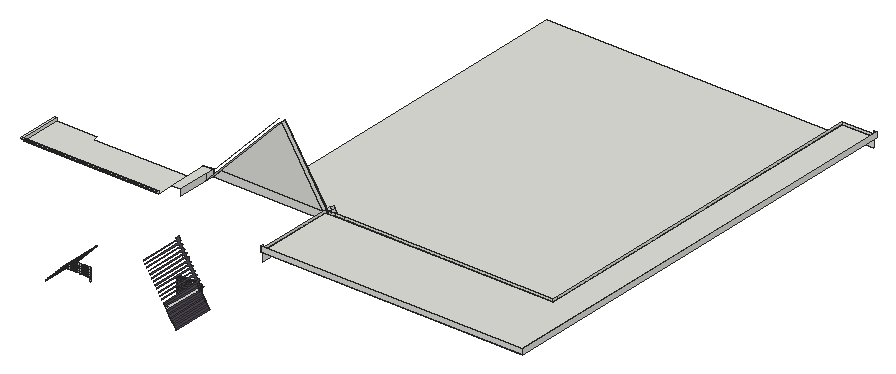
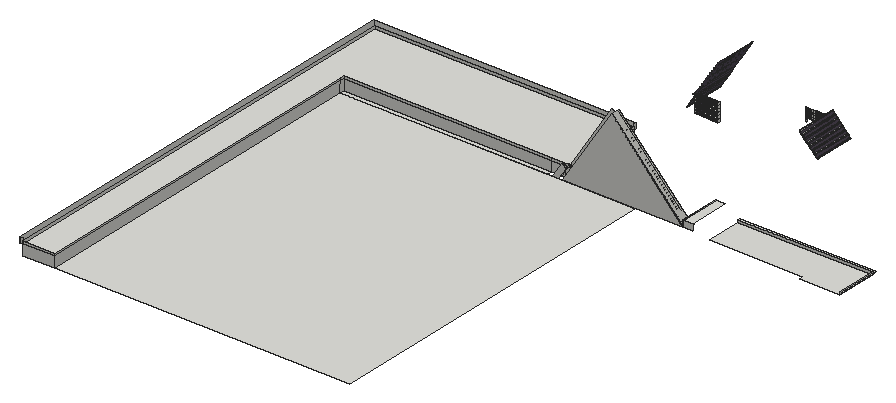
# SketchUp Ruby script. Lengths in inches.
U = 1.inch
M = Sketchup.active_model
def pt(a) = Geom::Point3d.new(a.map { |v| v * U })
def face(e, loops, mat)
  f = e.add_face(loops[0].map { |a| pt(a) })
  loops[1..].each { |l| e.add_face(l.map { |a| pt(a) }).erase! }
  f.material = f.back_material = mat if mat
  f
end
# faces: each face lists its corners as indices into pts; further lists are holes
def faces(e, pts, list, mat = nil) = list.each { |f| face(e, (f[0].is_a?(Array) ? f : [f]).map { |l| l.map { |i| pts[i] } }, mat) }
# xy, xz, yz: faces in a plane at the given z, y or x. An outline is a flat list of corners, or four numbers for a rectangle; further outlines are holes
def ring(l) = l.size == 4 ? [[l[0], l[1]], [l[2], l[1]], [l[2], l[3]], [l[0], l[3]]] : l.each_slice(2).to_a
def flat(e, list, mat, &to3) = list.each { |f| face(e, (f[0].is_a?(Array) ? f : [f]).map { |l| ring(l).map { |u, v| to3.(u, v) } }, mat) }
def xy(e, z, list, mat = nil) = flat(e, list, mat) { |x, y| [x, y, z] }
def xz(e, y, list, mat = nil) = flat(e, list, mat) { |x, z| [x, y, z] }
def yz(e, x, list, mat = nil) = flat(e, list, mat) { |y, z| [x, y, z] }
def lines(e, pts, list) = list.each { |a, b| e.add_line(pt(pts[a]), pt(pts[b])) }
# prism: a flat outline (further loops are holes) pulled along v
def prism(e, loops, v, mat = nil)
  f = face(e, loops, mat); d = Geom::Vector3d.new(v.map { |x| x * U })
  f.pushpull(f.normal.samedirection?(d) ? d.length : -d.length)
end
def box(e, o, s, mat = nil) = prism(e, [[o, [o[0] + s[0], o[1], o[2]], [o[0] + s[0], o[1] + s[1], o[2]], [o[0], o[1] + s[1], o[2]]]], [0, 0, s[2]], mat)
def at(x, y, z, deg = 0) = Geom::Transformation.translation(pt([x, y, z])) * Geom::Transformation.rotation(ORIGIN, Z_AXIS, deg.degrees)
def axes(o, x, y, z) = Geom::Transformation.new([*x, 0, *y, 0, *z, 0, *pt(o).to_a, 1])
def part(name) = M.definitions.add(name)
# library, detail: a bought-in or finely detailed component or shape, given as its bounding box
def library(name, o, s) = part(name).tap { |d| box(d.entities, o, s) }
def detail(e, o, s) = box(e.add_group.entities, o, s)
def put(e, d, t, mat = nil) = e.add_instance(d, t).tap { |i| i.material = mat if mat }
def group(e, t, mat = nil) = e.add_group.tap { |g| g.transformation = t; g.material = mat if mat }.entities
root = M.entities
M.materials.add("[Color M06]").color = [79, 71, 84]
xy(root,341.52,[[1096.79,2376.24,1127.76,2378.12]])
xy(root,341.93,[[1096.79,2376.24,1127.76,2378.12]])
xy(root,342.6875,[[771.375,2530.63,948.3125,2530.63,948.3125,2578.12,824.9375,2578.12,824.9375,2584.2,771.375,2584.2]])
xy(root,345.06,[[1096.79,2376.24,1127.76,2378.12]])
xy(root,346,[[1096.79,2376.24,1127.76,2378.12]])
xy(root,346.3125,[[768.8125,2528.07,771.375,2530.63],[771.375,2528.07,948.3125,2530.63],[768.8125,2530.63,771.375,2584.2]])
xy(root,349.12,[[1096.79,2376.24,1127.76,2378.12]])
xy(root,350.06,[[1096.79,2376.24,1127.76,2378.12]])
xy(root,350.1875,[[1156.15,2578.12,1429.3,2584.2],[1041.36,2584.2,1429.3,3053.87]])
xy(root,353.18,[[1096.79,2376.24,1127.76,2378.12]])
xy(root,354.12,[[1096.79,2376.24,1127.76,2378.12]])
xy(root,355.71,[[984.09,2332.13,986.27,2332.76],[986.875,2332.13,989.1875,2332.76],[989.79,2332.13,992.1,2332.76],[995.61,2332.13,997.92,2332.76],[1004.35,2332.13,1006.66,2332.76],
  [1007.26,2332.13,1009.57,2332.76],[1010.17,2332.13,1012.48,2332.76],[1013.08,2332.13,1015.4,2332.76],[1015.99,2332.13,1018.31,2332.76]])
xy(root,356.21,[[984.5625,2332.13,986.27,2332.76],[986.875,2332.13,989.1875,2332.76],[989.79,2332.13,992.1,2332.76],[992.7,2332.13,995.01,2332.76],[995.61,2332.13,997.92,2332.76],
  [998.52,2332.13,1000.83,2332.76],[1001.43,2332.13,1003.75,2332.76],[1004.35,2332.13,1006.66,2332.76],[1007.26,2332.13,1009.57,2332.76],[1010.17,2332.13,1012.48,2332.76],
  [1013.08,2332.13,1015.4,2332.76],[1015.99,2332.13,1018.31,2332.76]])
xy(root,357.25,[[1096.79,2376.24,1127.76,2378.12]])
xy(root,358.06,[[1096.79,2376.24,1127.76,2378.12]])
xy(root,358.5,[[965.61,2530.63,977.92,2584.2]])
xy(root,358.52,[[986.875,2332.13,989.1875,2332.76],[989.79,2332.13,992.1,2332.76],[992.7,2332.13,995.01,2332.76],[995.61,2332.13,997.92,2332.76],[998.52,2332.13,1000.83,2332.76],
  [1001.43,2332.13,1003.75,2332.76],[1004.35,2332.13,1006.66,2332.76],[1007.26,2332.13,1009.57,2332.76],[1010.17,2332.13,1012.48,2332.76],[1013.08,2332.13,1015.4,2332.76],
  [1015.99,2332.13,1018.31,2332.76]])
xy(root,359.02,[[987.2,2332.13,989.1875,2332.76],[989.79,2332.13,992.1,2332.76],[992.7,2332.13,995.01,2332.76],[995.61,2332.13,997.92,2332.76],[998.52,2332.13,1000.83,2332.76],
  [1001.43,2332.13,1003.75,2332.76],[1004.35,2332.13,1006.66,2332.76],[1007.26,2332.13,1009.57,2332.76],[1010.17,2332.13,1012.48,2332.76],[1013.08,2332.13,1015.4,2332.76],
  [1015.99,2332.13,1018.31,2332.76]])
xy(root,361.18,[[1096.79,2376.24,1127.76,2378.12]])
xy(root,361.34,[[989.79,2332.13,992.1,2332.76],[992.7,2332.13,995.01,2332.76],[995.61,2332.13,997.92,2332.76],[998.52,2332.13,1000.83,2332.76],[1001.43,2332.13,1003.75,2332.76],
  [1004.35,2332.13,1006.66,2332.76],[1007.26,2332.13,1009.57,2332.76],[1010.17,2332.13,1012.48,2332.76],[1013.08,2332.13,1015.4,2332.76],[1015.99,2332.13,1018.31,2332.76]])
xy(root,361.84,[[989.84,2332.13,992.1,2332.76],[992.7,2332.13,995.01,2332.76],[995.61,2332.13,997.92,2332.76],[998.52,2332.13,1000.83,2332.76],[1001.43,2332.13,1003.75,2332.76],
  [1004.35,2332.13,1006.66,2332.76],[1007.26,2332.13,1009.57,2332.76],[1010.17,2332.13,1012.48,2332.76],[1013.08,2332.13,1015.4,2332.76],[1015.99,2332.13,1018.31,2332.76]])
xy(root,362,[[1096.79,2376.24,1127.76,2378.12]])
xy(root,363.75,[[1130.09,2472.4,1470.74,2475.84],[1470.74,2472.4,1474.18,2475.84],[1130.09,2475.84,1130.09,2578.12,1429.3,2578.12,1429.3,3053.87,1470.74,3053.87,1470.74,2475.84],[1470.74,2475.84,1474.18,3053.87]])
xy(root,363.92,[[1127.76,2373.56,1129.63,2378.12]])
xy(root,364.15,[[992,2332.13,992.1,2332.76],[992.7,2332.13,995.01,2332.76],[995.61,2332.13,997.92,2332.76],[998.52,2332.13,1000.83,2332.76],[1001.43,2332.13,1003.75,2332.76],
  [1004.35,2332.13,1006.66,2332.76],[1007.26,2332.13,1009.57,2332.76],[1010.17,2332.13,1012.48,2332.76],[1013.08,2332.13,1015.4,2332.76],[1015.99,2332.13,1018.31,2332.76]])
xy(root,364.65,[[992.7,2332.13,995.01,2332.76],[995.61,2332.13,997.92,2332.76],[998.52,2332.13,1000.83,2332.76],[1001.43,2332.13,1003.75,2332.76],[1004.35,2332.13,1006.66,2332.76],
  [1007.26,2332.13,1009.57,2332.76],[1010.17,2332.13,1012.48,2332.76],[1013.08,2332.13,1015.4,2332.76],[1015.99,2332.13,1018.31,2332.76]])
xy(root,365.12,[[1096.79,2376.24,1126.98,2378.12]])
xz(root,2332.76,[[1015.99,350.59,1018.31,352.9],[1015.99,353.4,1018.31,355.71]])
xz(root,2371.68,[[1129.26,360.76,1129.63,360.99,1129.57,361.08,1129.21,360.85],[1128.57,361.83,1128.94,362.07,1127.76,363.92,1127.76,363.11],[1127.76,363.11,1127.39,363.68,1127.76,363.92],[1126.93,364.39,1126.88,364.48,1127.25,364.71,1127.3,364.625]])
xz(root,2373.56,[[970.79,341.69,973.21,344.27,972.75,344.7,970.33,342.125],[1140.21,343.68,1140.58,343.92,1138.88,346.56,1138.52,346.32],[974.08,345.2,976.51,347.77,976.05,348.2,973.63,345.63],[1137.88,347.3125,1138.25,347.55,1136.56,350.19,1136.1875,349.95],[977.38,348.7,979.8,351.28,979.35,351.7,976.93,349.13],
  [1135.56,350.94,1135.92,351.18,1134.23,353.82,1133.86,353.58],[980.68,352.21,983.1,354.78,982.65,355.21,980.23,352.64],[1133.23,354.57,1133.6,354.81,1131.9,357.45,1131.53,357.22],[983.98,355.71,986.4,358.28,985.95,358.71,983.53,356.14],[1130.9,358.2,1131.27,358.4375,1129.63,360.99,1129.63,360.18],
  [987.28,359.22,989.7,361.79,989.25,362.22,986.82,359.64],[1129.63,360.18,1129.26,360.76,1129.63,360.99],[1129.63,360.99,1129.63,363.92,1127.76,363.92,1128.94,362.07,1129.57,361.08],[990.58,362.72,993,365.29,992.54,365.72,990.12,363.15],[1127.39,363.68,1126.93,364.39,1127.3,364.625,1127.76,363.92],
  [1126.25,365.46,1124.61,368.02,1124.98,368.25,1126.61,365.7]])
xz(root,2376.24,[[1096.79,341.93,1127.76,345.06],[1096.79,346,1127.76,349.12],[1096.79,350.06,1127.76,353.18],[1096.79,354.12,1127.76,357.25],[1096.79,358.06,1127.76,361.18],
  [1096.79,362,1127.76,362,1127.76,363.92,1126.98,365.12,1096.79,365.12]],"[Color M06]")
xz(root,2378.12,[[1096.79,341.52,1127.76,341.93],[1096.79,345.06,1127.76,346],[1096.79,349.12,1127.76,350.06],[1096.79,353.18,1127.76,354.12],[1096.79,357.25,1127.76,358.06],
  [1096.79,361.18,1127.76,362],[1127.76,363.92,1127.76,365.12,1126.98,365.12],[1096.79,365.12,1126.98,365.12,1126.26,366.25,1096.79,366.25]])
xz(root,2472.4,[[1130.09,363.75,1474.18,370.8125]])
xz(root,2475.84,[[1130.09,363.75,1470.74,367.1875]])
xz(root,2530.63,[[771.375,342.6875,948.3125,346.3125]])
xz(root,2578.12,[[1130.09,350.1875,1130.09,360.28,1136.56,350.1875],[1136.56,350.1875,1136.56,359.1,1133.58,363.75,1130.09,363.75,1130.09,360.28],[1136.56,350.1875,1142.28,350.1875,1136.56,359.1],[1142.28,350.1875,1136.56,359.1,1136.56,363.75,1142.28,363.75],[1142.28,350.1875,1156.15,363.75],
  [1156.15,350.1875,1429.3,363.75],[1136.56,359.1,1133.58,363.75,1136.56,363.75],[1130.09,360.28,1130.09,364.9375,1127.1,364.9375],[1130.09,363.75,1130.09,364.9375,1132.82,364.9375,1133.58,363.75],[1133.58,363.75,1132.82,364.9375,1131.375,367.1875,1133.58,367.1875],
  [1133.58,363.75,1136.56,367.1875],[1136.56,363.75,1142.28,367.1875],[1142.28,363.75,1156.15,367.1875],[1156.15,363.75,1429.3,367.1875],[991.81,364.9375,1072.29,450.4375,1127.1,364.9375],
  [1127.1,364.9375,1072.29,450.4375,1076.34,453.03,1131.15,367.53,1130.61,367.1875,1130.09,367.1875,1130.09,366.85],[1127.1,364.9375,1130.09,366.85,1130.09,364.9375],[1130.09,364.9375,1130.09,366.85,1130.61,367.1875,1131.375,367.1875,1132.82,364.9375]])
xz(root,2583.74,[[965.61,357.04,964.88,357.73,965.61,358.5]])
xz(root,2584.2,[[1149.7,340.75,1153.99,343.5,1149.7,350.1875],[1142.28,341.27,1142.28,350.1875,1136.56,350.1875],[965.61,350.1875,977.92,358.5],[977.92,350.1875,1072.29,450.4375,1136.56,350.1875],[1142.28,350.1875,1132.82,364.9375,1138.08,368.3125,1149.7,350.1875],
  [1132.82,364.9375,1131.15,367.53,1136.41,370.91,1138.08,368.3125]])
xz(root,3053.87,[[1429.3,350.1875,1470.74,363.75],[1429.3,363.75,1470.74,367.1875],[1470.74,363.75,1474.18,370.8125]])
yz(root,771.375,[[2530.63,342.6875,2584.2,346.3125]])
yz(root,977.92,[[2530.63,350.1875,2571.59,358.5],[2571.59,350.1875,2583.74,358.5],[2583.74,350.1875,2584.2,358.5]])
yz(root,986.27,[[2332.13,356.21,2332.76,358.04]])
yz(root,986.875,[[2332.13,356.21,2332.76,358.52]])
yz(root,989.1875,[[2332.13,356.21,2332.76,358.52],[2332.13,359.02,2332.76,361.14]])
yz(root,989.79,[[2332.13,356.21,2332.76,358.52],[2332.13,359.02,2332.76,361.34]])
yz(root,992.1,[[2332.13,356.21,2332.76,358.52],[2332.13,359.02,2332.76,361.34],[2332.13,361.84,2332.76,364.15]])
yz(root,992.7,[[2332.13,356.21,2332.76,358.52],[2332.13,359.02,2332.76,361.34],[2332.13,361.84,2332.76,364.15],[2332.13,364.65,2332.76,364.89]])
yz(root,995.01,[[2332.13,356.21,2332.76,358.52],[2332.13,359.02,2332.76,361.34],[2332.13,361.84,2332.76,364.15],[2332.13,364.65,2332.76,366.96]])
yz(root,995.61,[[2332.13,356.21,2332.76,358.52],[2332.13,359.02,2332.76,361.34],[2332.13,361.84,2332.76,364.15],[2332.13,364.65,2332.76,366.96]])
yz(root,997.92,[[2332.13,356.21,2332.76,358.52],[2332.13,359.02,2332.76,361.34],[2332.13,361.84,2332.76,364.15],[2332.13,364.65,2332.76,366.96]])
yz(root,998.52,[[2332.13,356.21,2332.76,358.52],[2332.13,359.02,2332.76,361.34],[2332.13,361.84,2332.76,364.15],[2332.13,364.65,2332.76,366.96]])
yz(root,1000.83,[[2332.13,356.21,2332.76,358.52],[2332.13,359.02,2332.76,361.34],[2332.13,361.84,2332.76,364.15],[2332.13,364.65,2332.76,366.96]])
yz(root,1001.43,[[2332.13,356.21,2332.76,358.52],[2332.13,359.02,2332.76,361.34],[2332.13,361.84,2332.76,364.15],[2332.13,364.65,2332.76,366.96]])
yz(root,1003.75,[[2332.13,356.21,2332.76,358.52],[2332.13,359.02,2332.76,361.34],[2332.13,361.84,2332.76,364.15],[2332.13,364.65,2332.76,366.96]])
yz(root,1004.35,[[2332.13,356.21,2332.76,358.52],[2332.13,359.02,2332.76,361.34],[2332.13,361.84,2332.76,364.15],[2332.13,364.65,2332.76,366.96]])
yz(root,1006.66,[[2332.13,356.21,2332.76,358.52],[2332.13,359.02,2332.76,361.34],[2332.13,361.84,2332.76,364.15],[2332.13,364.65,2332.76,366.96]])
yz(root,1007.26,[[2332.13,356.21,2332.76,358.52],[2332.13,359.02,2332.76,361.34],[2332.13,361.84,2332.76,364.15],[2332.13,364.65,2332.76,366.96]])
yz(root,1009.57,[[2332.13,356.21,2332.76,358.52],[2332.13,359.02,2332.76,361.34],[2332.13,361.84,2332.76,364.15],[2332.13,364.65,2332.76,366.96]])
yz(root,1010.17,[[2332.13,356.21,2332.76,358.52],[2332.13,359.02,2332.76,361.34],[2332.13,361.84,2332.76,364.15],[2332.13,364.65,2332.76,366.96]])
yz(root,1012.48,[[2332.13,356.21,2332.76,358.52],[2332.13,359.02,2332.76,361.34],[2332.13,361.84,2332.76,364.15],[2332.13,364.65,2332.76,366.96]])
yz(root,1013.08,[[2332.13,356.21,2332.76,358.52],[2332.13,359.02,2332.76,361.34],[2332.13,361.84,2332.76,364.15],[2332.13,364.65,2332.76,366.96]])
yz(root,1015.4,[[2332.13,356.21,2332.76,358.52],[2332.13,359.02,2332.76,361.34],[2332.13,361.84,2332.76,364.15],[2332.13,364.65,2332.76,366.96]])
yz(root,1015.99,[[2332.13,356.21,2332.76,358.52],[2332.13,359.02,2332.76,361.34],[2332.13,361.84,2332.76,364.15],[2332.13,364.65,2332.76,366.96]])
yz(root,1018.31,[[2332.13,356.21,2332.76,358.52],[2332.13,359.02,2332.76,361.34],[2332.13,361.84,2332.76,364.15],[2332.13,364.65,2332.76,366.96]])
yz(root,1096.79,[[2376.24,341.93,2378.12,345.06],[2376.24,346,2378.12,349.12],[2376.24,350.06,2378.12,353.18],[2376.24,354.12,2378.12,357.25],[2376.24,358.06,2378.12,361.18],
  [2376.24,362,2378.12,365.12]])
yz(root,1127.76,[[2376.24,341.93,2378.12,345.06],[2376.24,346,2378.12,349.12],[2376.24,350.06,2378.12,353.18],[2376.24,354.12,2378.12,357.25],[2376.24,358.06,2378.12,361.18],
  [2376.24,362,2378.12,363.92]])
yz(root,1130.09,[[2475.84,350.1875,2578.12,363.75],[2472.4,363.75,2475.84,370.8125],[2475.84,363.75,2578.12,367.1875]])
yz(root,1429.3,[[2578.12,350.1875,2584.2,363.75],[2584.2,350.1875,3053.87,363.75],[2578.12,363.75,2584.2,367.1875],[2584.2,363.75,3053.87,367.1875]])
yz(root,1470.74,[[2475.84,363.75,3053.87,367.1875]])
yz(root,1474.18,[[2472.4,363.75,3053.87,370.8125]])
p = [[969.45,2373.56,341.19],[969.45,2319.18,341.19],[969.91,2319.18,340.76],[969.91,2373.56,340.76],[970.33,2373.56,342.125],[970.33,2319.18,342.125],
  [970.79,2373.56,341.69],[970.79,2319.18,341.69],[973.21,2373.56,344.27],[973.21,2319.18,344.27],[1141.21,2319.18,342.93],[1141.21,2373.56,342.93],
  [1140.84,2373.56,342.69],[1140.84,2319.18,342.69],[1140.58,2319.18,343.92],[1140.58,2373.56,343.92],[1138.52,2373.56,346.32],[1140.21,2373.56,343.68],
  [1140.21,2319.18,343.68],[1138.52,2319.18,346.32],[972.75,2373.56,344.7],[972.75,2319.18,344.7],[973.63,2373.56,345.63],[973.63,2319.18,345.63],
  [974.08,2373.56,345.2],[974.08,2319.18,345.2],[976.51,2373.56,347.77],[976.51,2319.18,347.77],[1138.88,2319.18,346.56],[1138.88,2373.56,346.56],
  [1138.25,2319.18,347.55],[1138.25,2373.56,347.55],[1136.1875,2373.56,349.95],[1137.88,2373.56,347.3125],[1137.88,2319.18,347.3125],[1136.1875,2319.18,349.95],
  [976.05,2373.56,348.2],[976.05,2319.18,348.2],[976.93,2373.56,349.13],[976.93,2319.18,349.13],[977.38,2373.56,348.7],[977.38,2319.18,348.7],
  [979.8,2373.56,351.28],[979.8,2319.18,351.28],[1136.56,2319.18,350.19],[1136.56,2373.56,350.19],[1135.92,2319.18,351.18],[1135.92,2373.56,351.18],
  [1072.29,2583.74,450.4375],[977.92,2583.74,350.1875],[977.92,2571.59,350.1875],[1072.29,2571.59,450.4375],[1072.29,2578.12,450.4375],[1072.29,2584.2,450.4375],
  [977.92,2584.2,350.1875],[1133.86,2373.56,353.58],[1135.56,2373.56,350.94],[1135.56,2319.18,350.94],[1133.86,2319.18,353.58],[979.35,2373.56,351.7],
  [979.35,2319.18,351.7],[980.23,2373.56,352.64],[980.23,2319.18,352.64],[980.68,2373.56,352.21],[980.68,2319.18,352.21],[983.1,2373.56,354.78],
  [983.1,2319.18,354.78],[1134.23,2319.18,353.82],[1134.23,2373.56,353.82],[1133.6,2319.18,354.81],[1133.6,2373.56,354.81],[1131.53,2373.56,357.22],
  [1133.23,2373.56,354.57],[1133.23,2319.18,354.57],[1131.53,2319.18,357.22],[982.65,2373.56,355.21],[982.65,2319.18,355.21],[983.53,2373.56,356.14],
  [983.53,2319.18,356.14],[983.98,2373.56,355.71],[983.98,2332.13,355.71],[983.98,2319.18,355.71],[986.4,2373.56,358.28],[986.4,2319.18,358.28],
  [986.27,2332.13,358.04],[984.5625,2332.13,356.21],[984.5625,2332.76,356.21],[986.27,2332.76,358.04],[1131.9,2319.18,357.45],[1131.9,2373.56,357.45],
  [1131.27,2319.18,358.4375],[1131.27,2373.56,358.4375],[1129.21,2319.18,360.85],[1129.21,2371.68,360.85],[1129.26,2371.68,360.76],[1129.26,2373.56,360.76],
  [1129.63,2373.56,360.18],[1130.9,2373.56,358.2],[1130.9,2319.18,358.2],[985.95,2373.56,358.71],[985.95,2319.18,358.71],[986.82,2373.56,359.64],
  [986.82,2319.18,359.64],[989.1875,2332.13,361.14],[987.2,2332.13,359.02],[987.2,2332.76,359.02],[989.1875,2332.76,361.14],[987.28,2373.56,359.22],
  [987.28,2319.18,359.22],[989.7,2373.56,361.79],[989.7,2319.18,361.79],[1129.57,2319.18,361.08],[1129.57,2371.68,361.08],[1129.63,2371.68,360.99],
  [1129.63,2373.56,360.99],[1129.57,2373.56,361.08],[1128.94,2319.18,362.07],[1128.94,2371.68,362.07],[1128.94,2373.56,362.07],[989.25,2373.56,362.22],
  [989.25,2319.18,362.22],[1126.88,2319.18,364.48],[1126.88,2371.68,364.48],[1126.93,2371.68,364.39],[1126.93,2373.56,364.39],[1127.39,2373.56,363.68],
  [1127.39,2371.68,363.68],[1127.76,2371.68,363.11],[1128.57,2371.68,361.83],[1128.57,2319.18,361.83],[992,2332.13,364.15],[989.84,2332.13,361.84],
  [989.84,2332.76,361.84],[992,2332.76,364.15],[1127.25,2319.18,364.71],[1127.25,2371.68,364.71],[1127.25,2373.56,364.71],[1127.3,2373.56,364.625],
  [1127.76,2373.56,363.92],[1127.76,2371.68,363.92],[990.12,2373.56,363.15],[990.12,2319.18,363.15],[990.58,2373.56,362.72],[990.58,2319.18,362.72],
  [993,2373.56,365.29],[993,2319.18,365.29],[1127.76,2376.24,363.92],[1126.61,2319.18,365.7],[1126.61,2373.56,365.7],[1124.98,2373.56,368.25],
  [1124.98,2371.68,368.25],[1124.92,2371.68,368.34],[1124.92,2319.18,368.34],[1124.29,2319.18,369.33],[1124.29,2373.56,369.33],[1122.65,2373.56,371.88],
  [1122.65,2371.68,371.88],[1122.59,2371.68,371.97],[1122.59,2319.18,371.97],[1122.09,2319.18,372.75],[1122.09,2373.56,372.75],[1120.46,2373.56,375.3],
  [1120.46,2371.68,375.3],[1120.4,2371.68,375.39],[1120.4,2319.18,375.39],[1119.9,2319.18,376.17],[1119.9,2373.56,376.17],[1118.26,2373.56,378.72],
  [1118.26,2371.68,378.72],[1118.21,2371.68,378.8125],[1118.21,2319.18,378.8125],[1117.71,2319.18,379.59],[1117.71,2373.56,379.59],[1116.07,2373.56,382.14],
  [1116.07,2371.68,382.14],[1116.01,2371.68,382.23],[1116.01,2319.18,382.23],[1115.52,2319.18,383.01],[1115.52,2373.56,383.01],[1113.88,2373.56,385.56],
  [1113.88,2371.68,385.56],[1113.82,2371.68,385.65],[1113.82,2319.18,385.65],[1113.32,2319.18,386.43],[1113.32,2373.56,386.43],[1111.69,2373.56,388.98],
  [1111.69,2371.68,388.98],[1111.63,2371.68,389.07],[1111.63,2319.18,389.07],[1111.13,2319.18,389.85],[1111.13,2373.56,389.85],[1109.49,2373.56,392.4],
  [1109.49,2371.68,392.4],[1109.4375,2371.68,392.49],[1109.4375,2319.18,392.49],[1108.9375,2319.18,393.27],[1108.9375,2373.56,393.27],[1107.3,2373.56,395.82],
  [1107.3,2371.68,395.82],[1107.24,2371.68,395.91],[1107.24,2319.18,395.91],[1106.75,2319.18,396.69],[1106.75,2373.56,396.69],[1105.11,2373.56,399.24],
  [1105.11,2371.68,399.24],[1105.05,2371.68,399.33],[1105.05,2319.18,399.33],[1104.55,2319.18,400.11],[1104.55,2373.56,400.11],[1102.91,2373.56,402.66],
  [1102.91,2371.68,402.66],[1102.86,2371.68,402.75],[1102.86,2319.18,402.75],[1102.36,2319.18,403.53],[1102.36,2373.56,403.53],[1100.72,2373.56,406.08],
  [1100.72,2371.68,406.08],[1100.67,2371.68,406.17],[1100.67,2319.18,406.17],[1100.17,2319.18,406.95],[1100.17,2373.56,406.95],[1098.53,2373.56,409.5],
  [1098.53,2371.68,409.5],[1098.47,2371.68,409.59],[1098.47,2319.18,409.59],[1097.97,2319.18,410.37],[1097.97,2373.56,410.37],[1096.79,2373.56,412.22],
  [1096.79,2378.12,412.22],[1096.85,2378.12,412.12],[1098.86,2378.12,409],[1099.74,2378.12,407.62],[1099.74,2376.24,407.62],[1101.74,2376.24,404.5],
  [1101.74,2378.12,404.5],[1102.46,2378.12,403.37],[1102.46,2376.24,403.37],[1104.47,2376.24,400.25],[1104.47,2378.12,400.25],[1105.1875,2378.12,399.12],
  [1105.1875,2376.24,399.12],[1107.19,2376.24,396],[1107.19,2378.12,396],[1107.91,2378.12,394.87],[1107.91,2376.24,394.87],[1109.92,2376.24,391.75],
  [1109.92,2378.12,391.75],[1110.64,2378.12,390.62],[1110.64,2376.24,390.62],[1112.64,2376.24,387.5],[1112.64,2378.12,387.5],[1113.36,2378.12,386.37],
  [1113.36,2376.24,386.37],[1115.36,2376.24,383.25],[1115.36,2378.12,383.25],[1116.08,2378.12,382.12],[1116.08,2376.24,382.12],[1118.09,2376.24,379],
  [1118.09,2378.12,379],[1118.81,2378.12,377.87],[1118.81,2376.24,377.87],[1120.8125,2376.24,374.75],[1120.8125,2378.12,374.75],[1121.53,2378.12,373.62],
  [1121.53,2376.24,373.62],[1123.54,2376.24,370.5],[1123.54,2378.12,370.5],[1124.26,2378.12,369.37],[1124.26,2376.24,369.37],[1126.26,2376.24,366.25],
  [1126.26,2378.12,366.25],[1126.98,2378.12,365.12],[1126.98,2376.24,365.12],[1127.76,2378.12,363.92],[1127.3,2371.68,364.625],[994.64,2332.13,366.96],
  [992.7,2332.13,364.89],[992.7,2332.76,364.89],[994.64,2332.76,366.96],[1131.375,2578.12,367.1875],[1131.15,2578.12,367.53],[1131.15,2584.2,367.53],
  [1132.82,2584.2,364.9375],[1132.82,2578.12,364.9375],[992.54,2373.56,365.72],[992.54,2319.18,365.72],[1124.55,2319.18,368.11],[1124.55,2371.68,368.11],
  [1124.61,2371.68,368.02],[1124.61,2373.56,368.02],[1126.25,2373.56,365.46],[1126.25,2319.18,365.46],[993.42,2373.56,366.65],[993.42,2319.18,366.65],
  [965.61,2583.74,358.5],[966.34,2583.74,357.81],[985.88,2578.12,364.9375],[1069.09,2578.12,453.34]]
faces(root,p,[[0,1,2,3],[10,11,12,13],[15,14,18,17],[23,22,24,25],[28,29,16,19],[31,30,34,33],[39,38,40,41],[44,45,32,35],
  [48,49,50,51,52],[53,54,49,48],[47,46,57,56],[62,61,63,64],[67,68,55,58],[70,69,73,72],[78,77,79,80,81],[84,85,86,87],
  [88,89,71,74],[91,90,98,97],[103,104,105,106],[102,101,107,108],[111,112,93,92],[113,114,95,94],[113,112,115,114],[112,117,118,115],
  [117,116,129,128],[130,131,132,133],[116,134,135,136,137,138,139,117],[138,118,117,139],[141,140,142,143],[138,139,126,125],[271,273,146,272],[274,137,124,123],
  [134,135,122,121],[275,276,277,278],[279,280,281,282,283],[284,285,145,144],[148,147,291,290]])
faces(root,p,[[0,4,5,1],[5,4,6,7],[6,8,9,7],[10,14,15,11],[16,17,18,19],[20,21,9,8],[20,22,23,21],[24,26,27,25],
  [28,30,31,29],[32,33,34,35],[36,37,27,26],[36,38,39,37],[40,42,43,41],[44,46,47,45],[55,56,57,58],[59,60,43,42],
  [59,61,62,60],[63,65,66,64],[67,69,70,68],[71,72,73,74],[75,76,66,65],[75,77,78,76],[79,82,83,81,80],[88,90,91,89],
  [92,93,94,95,96,97,98],[99,100,83,82],[99,101,102,100],[107,109,110,108],[111,116,117,112],[119,120,110,109],[121,122,123,124,125,126,127,128,129],[119,140,141,120],
  [142,144,145,143],[146,138,137,136,135,134,147,148,149,150,151,152,153,154,155,156,157,158,159,160,161,162,163,164,165,166,167,168,169,170,171,172,173,174,175,176,177,178,179,180,181,182,183,184,185,186,187,188,189,190,191,192,193,194,195,196,197,198,199,200,201,202,203,204,205,206,207,208,209,210,211,212,213,214,215,216,217,218,219,220,221,222,223,224,225,226,227,228,229,230,231,232,233,234,235,236,237,238,239,240,241,242,243,244,245,246,247,248,249,250,251,252,253,254,255,256,257,258,259,260,261,262,263,264,265,266,267,268,269,270,271,272],[286,287,288,289,290,291],[284,292,293,285]],"[Color M06]")
lines(root,p,[[294,295],[296,297]])
